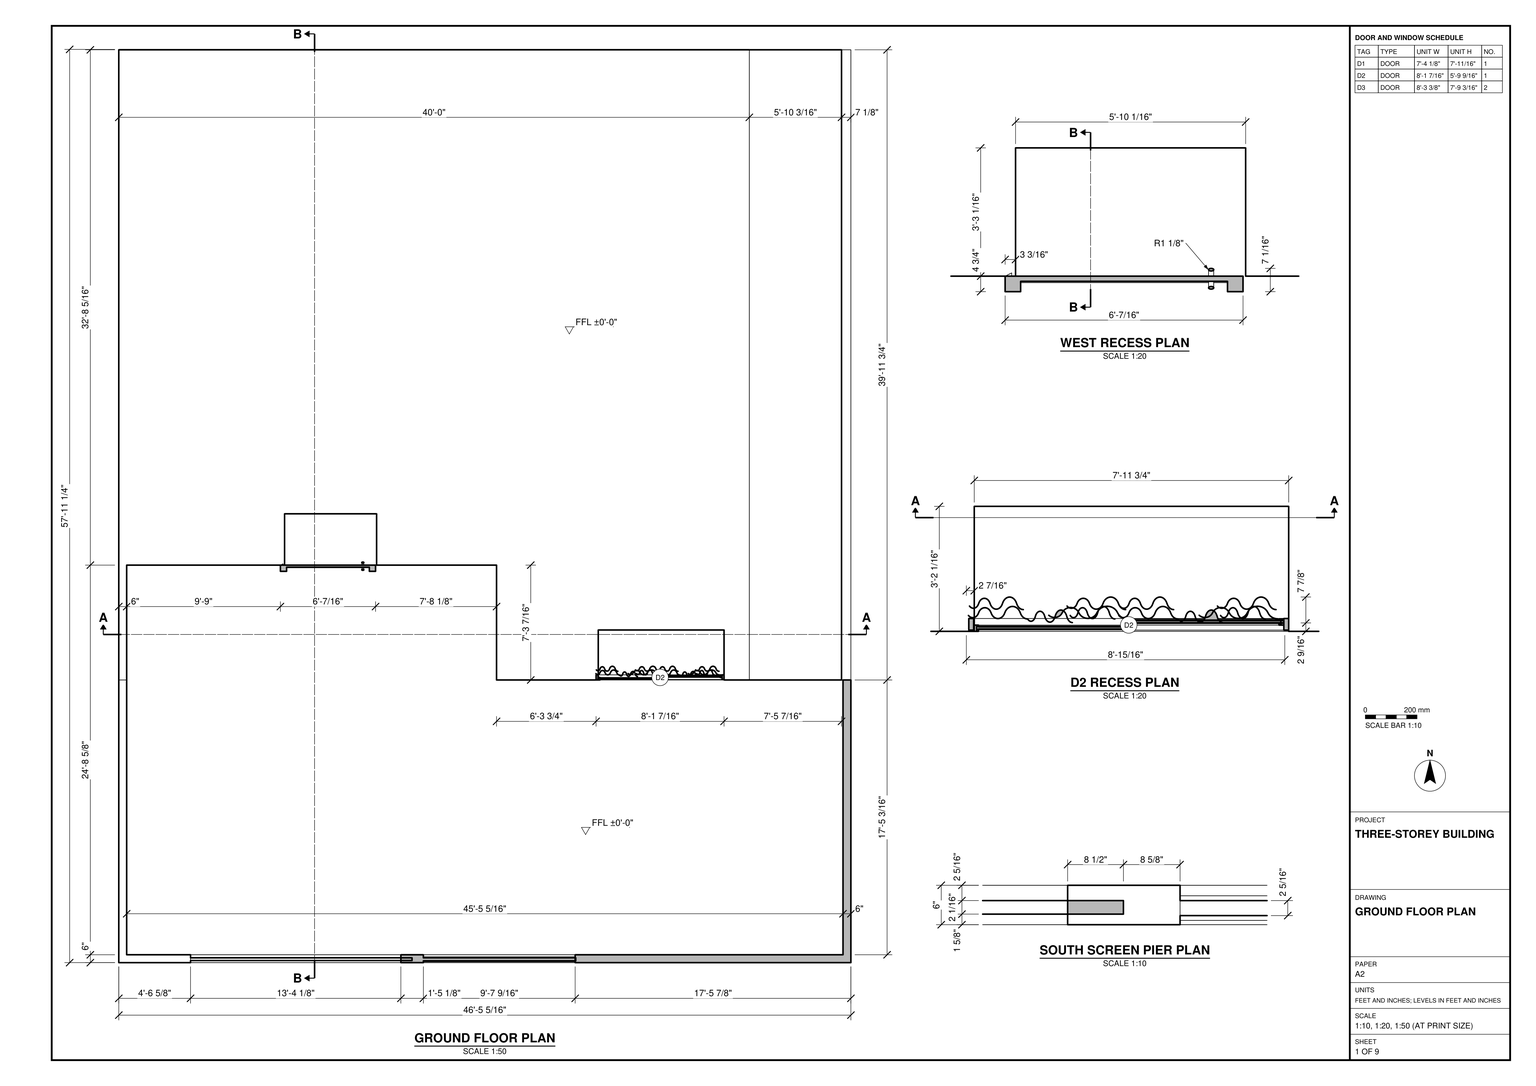
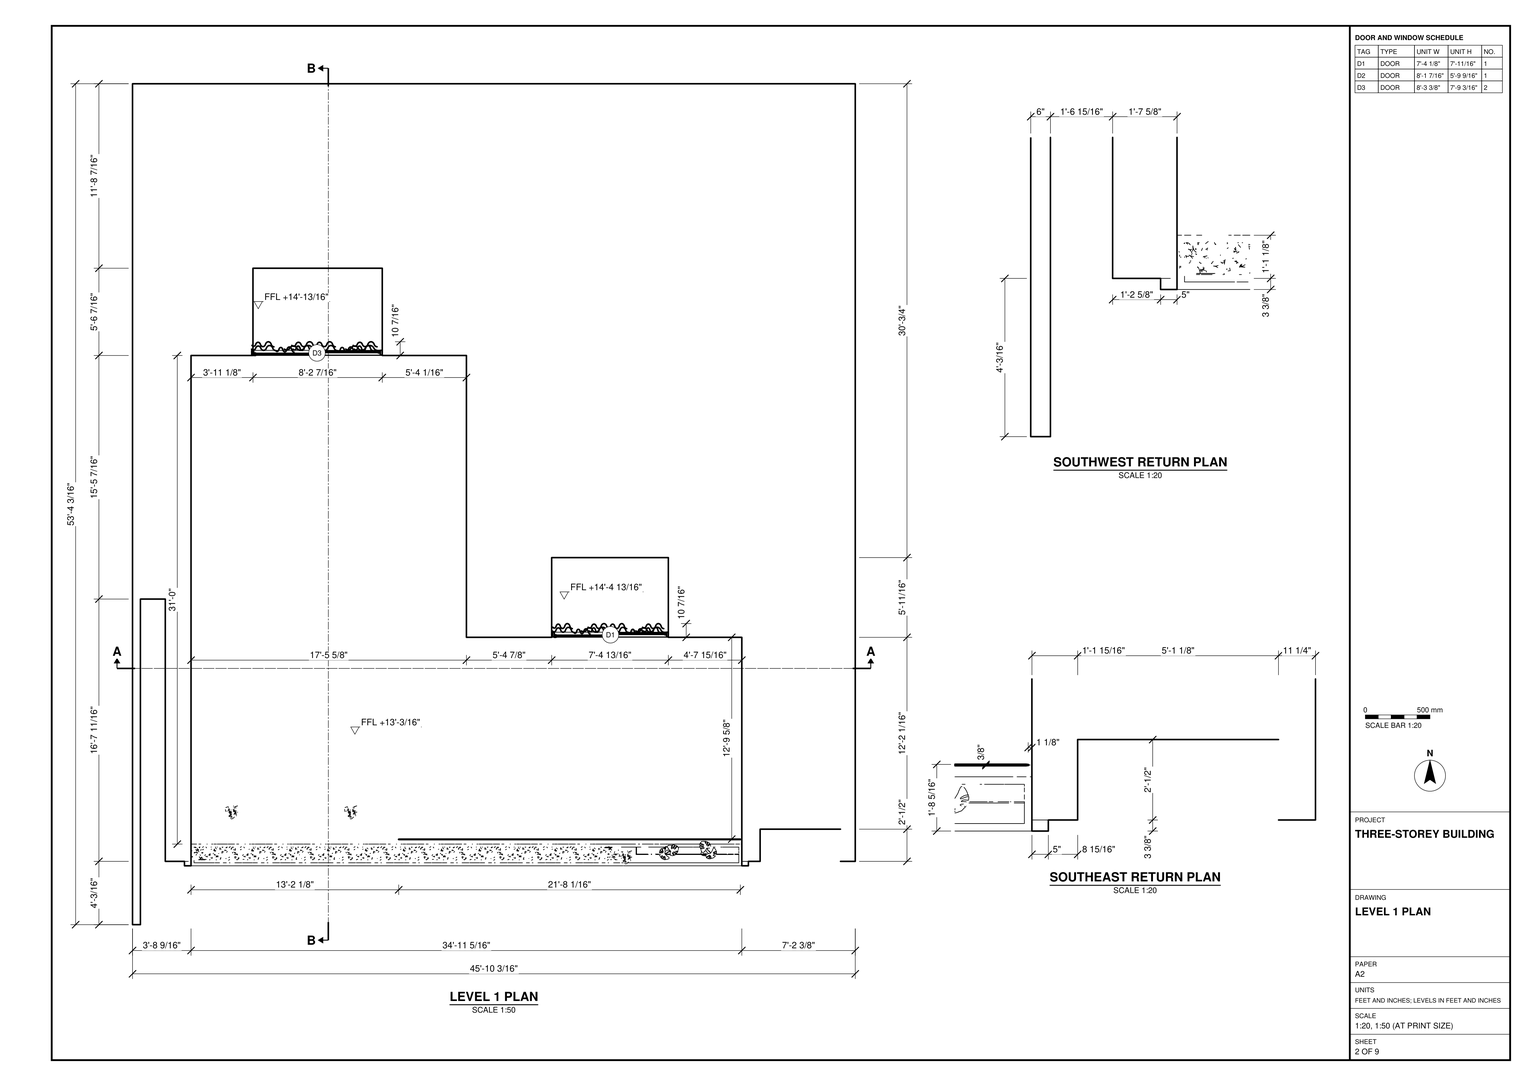
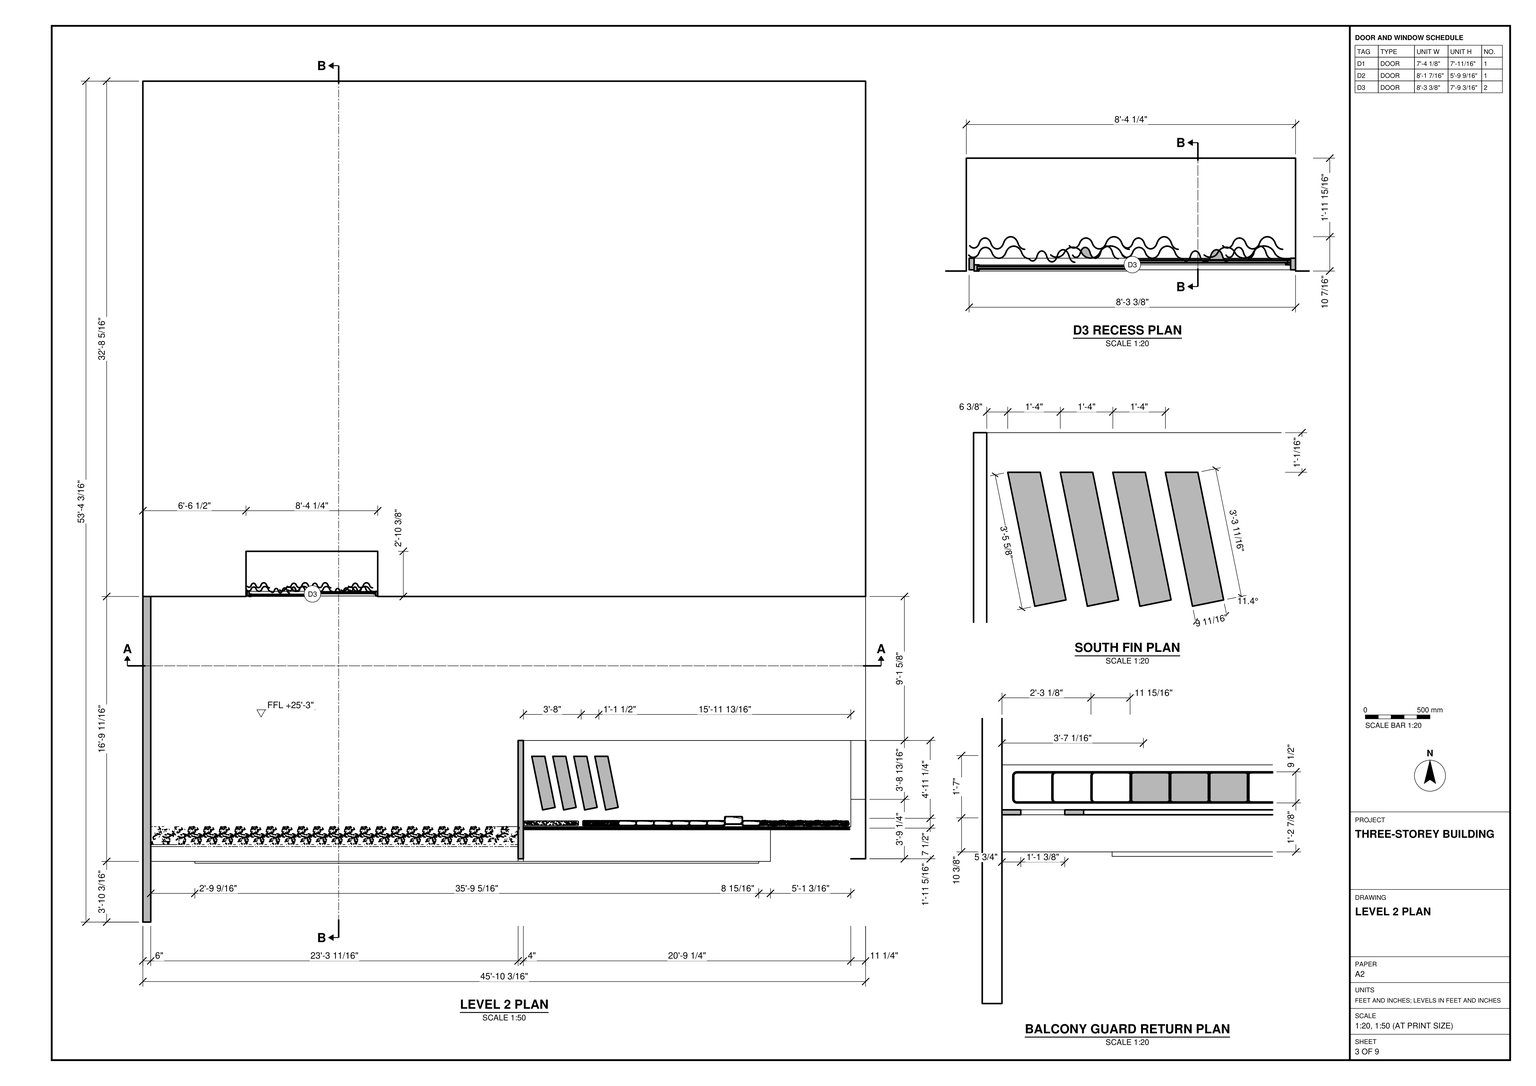
Build the three-storey building shown in task_files/diagram_01.pdf. Work in feet and inches in SketchUp. Orient the model so that the south frontage runs along the X axis. The overall dimensions are 46'-5 5/16" east to west, 57'-11 1/4" north to south and 35'-10 3/8" high. Set the ground floor at ±0'-0", level 1 at +13'-3/16" and level 2 at +25'-3".

Use each floor plan to set out its own walls and slab edges. Follow the wall thicknesses, changes in depth and projecting returns shown on that plan. Complete the roof to the profile shown on the sheets. On the ground floor, distinguish the west recess from the recessed glazed door farther east, and include the pier between the south screen spans. On level 1, place the recessed doors on their respective faces of the stepped wall. Use the enlarged details for the door frames, balcony guards and wall returns. On level 2, include the planting along the south balcony and the angled fins beside the dividing wall.

Keep shell elements such as walls, slabs and roof, and each furniture or joinery piece shown, in separate groups or components. Use components for repeated parts. Decor and loose items, including plants, may be any suitable library components. Save one SketchUp model as output_files/three_storey_building_with_south_balconies.skp.

# SketchUp Ruby script. Lengths in inches.
U = 1.inch
M = Sketchup.active_model
def pt(a) = Geom::Point3d.new(a.map { |v| v * U })
def face(e, loops, mat)
  f = e.add_face(loops[0].map { |a| pt(a) })
  loops[1..].each { |l| e.add_face(l.map { |a| pt(a) }).erase! }
  f.material = f.back_material = mat if mat
  f
end
# faces: each face lists its corners as indices into pts; further lists are holes
def faces(e, pts, list, mat = nil) = list.each { |f| face(e, (f[0].is_a?(Array) ? f : [f]).map { |l| l.map { |i| pts[i] } }, mat) }
# xy, xz, yz: faces in a plane at the given z, y or x. An outline is a flat list of corners, or four numbers for a rectangle; further outlines are holes
def ring(l) = l.size == 4 ? [[l[0], l[1]], [l[2], l[1]], [l[2], l[3]], [l[0], l[3]]] : l.each_slice(2).to_a
def flat(e, list, mat, &to3) = list.each { |f| face(e, (f[0].is_a?(Array) ? f : [f]).map { |l| ring(l).map { |u, v| to3.(u, v) } }, mat) }
def xy(e, z, list, mat = nil) = flat(e, list, mat) { |x, y| [x, y, z] }
def xz(e, y, list, mat = nil) = flat(e, list, mat) { |x, z| [x, y, z] }
def yz(e, x, list, mat = nil) = flat(e, list, mat) { |y, z| [x, y, z] }
def lines(e, pts, list) = list.each { |a, b| e.add_line(pt(pts[a]), pt(pts[b])) }
# prism: a flat outline (further loops are holes) pulled along v
def prism(e, loops, v, mat = nil)
  f = face(e, loops, mat); d = Geom::Vector3d.new(v.map { |x| x * U })
  f.pushpull(f.normal.samedirection?(d) ? d.length : -d.length)
end
def box(e, o, s, mat = nil) = prism(e, [[o, [o[0] + s[0], o[1], o[2]], [o[0] + s[0], o[1] + s[1], o[2]], [o[0], o[1] + s[1], o[2]]]], [0, 0, s[2]], mat)
def at(x, y, z, deg = 0) = Geom::Transformation.translation(pt([x, y, z])) * Geom::Transformation.rotation(ORIGIN, Z_AXIS, deg.degrees)
def axes(o, x, y, z) = Geom::Transformation.new([*x, 0, *y, 0, *z, 0, *pt(o).to_a, 1])
def part(name) = M.definitions.add(name)
# library, detail: a bought-in or finely detailed component or shape, given as its bounding box
def library(name, o, s) = part(name).tap { |d| box(d.entities, o, s) }
def detail(e, o, s) = box(e.add_group.entities, o, s)
def put(e, d, t, mat = nil) = e.add_instance(d, t).tap { |i| i.material = mat if mat }
def group(e, t, mat = nil) = e.add_group.tap { |g| g.transformation = t; g.material = mat if mat }.entities
root = M.entities
M.materials.add("Color_004").color = [142, 142, 142]
M.materials.add("Material__1").color = [51, 42, 44]
M.materials.add("Material__2").color = [97, 132, 37]
M.materials.add("Painted Metal Railing").color = [35, 35, 35]
M.materials.add("Teddy_Paper").color = [237, 237, 189]
M.materials.add("[0135_DarkGray]").color = [81, 81, 81]
M.materials.add("[Color_007]").color = [58, 58, 58]
M.materials.add("[Translucent_Glass_Gray] copy").color = [139, 139, 139]
M.materials["[Translucent_Glass_Gray] copy"].alpha = 0.15
M.materials.add("[Wood Lumber ButtJoined]").color = [164, 152, 112]
M.materials.add("[Wood Veneer 01]1").color = [120, 70, 37]
c1 = part("Post")
box(c1.entities,[-0.75,-0.75,0],[1.5,1.5,34.5],"Painted Metal Railing")
c2 = part("Group43\#1")
box(c2.entities,[-0.75,0,0],[1.5,73.5,1.5],"Painted Metal Railing")
c3 = part("Group46\#2")
box(c3.entities,[-0.75,0.75,0],[1.5,34.5,1.5],"Painted Metal Railing")
c4 = part("Group49\#1")
box(c4.entities,[-0.75,0.75,0],[1.5,34.5,1.5],"Painted Metal Railing")
c5 = part("Group52\#1")
box(c5.entities,[-0.75,0.75,0],[1.5,34.5,1.5],"Painted Metal Railing")
c6 = part("Group55\#1")
box(c6.entities,[-0.75,0.75,0],[1.5,34.5,1.5],"Painted Metal Railing")
c7 = part("Inner Post")
box(c7.entities,[-0.75,-0.75,0],[1.5,1.5,23.5],"Painted Metal Railing")
c8 = part("Group59\#1")
box(c8.entities,[-0.75,0.75,0],[1.5,24.5,1.5],"Painted Metal Railing")
c9 = part("Group62\#1")
box(c9.entities,[-0.75,0.75,0],[1.5,24.5,1.5],"Painted Metal Railing")
c10 = part("Group65\#1")
box(c10.entities,[-0.75,0.75,0],[1.5,24.5,1.5],"Painted Metal Railing")
c11 = part("Inner Posts and Rails\#2")
put(c11.entities,c7,at(0,0,0,90))
put(c11.entities,c7,at(0,26,0,90))
put(c11.entities,c8,at(0,0,4.75))
put(c11.entities,c9,at(0,0,11))
put(c11.entities,c10,at(0,0,17.25))
c12 = part("Group69\#1")
box(c12.entities,[-0.75,0.75,0],[1.5,24.5,1.5],"Painted Metal Railing")
c13 = part("Group72\#1")
box(c13.entities,[-0.75,0.75,0],[1.5,24.5,1.5],"Painted Metal Railing")
c14 = part("Group75\#1")
box(c14.entities,[-0.75,0.75,0],[1.5,24.5,1.5],"Painted Metal Railing")
c15 = part("Inner Posts and Rails\#3")
put(c15.entities,c7,at(0,0,0,90))
put(c15.entities,c7,at(0,26,0,90))
put(c15.entities,c12,at(0,0,4.75))
put(c15.entities,c13,at(0,0,11))
put(c15.entities,c14,at(0,0,17.25))
c16 = part("Railing Assembly 14\#1")
put(c16.entities,c1,at(0,0,0))
put(c16.entities,c1,at(36,0,0))
put(c16.entities,c1,at(72,0,0))
put(c16.entities,c2,at(-0.75,0,34.5,-90))
put(c16.entities,c3,at(0,0,4,-90))
put(c16.entities,c4,at(36,0,4,-90))
put(c16.entities,c5,at(0,0,29,-90))
put(c16.entities,c6,at(36,0,29,-90))
put(c16.entities,c11,at(5,0,5.5,-90))
put(c16.entities,c15,at(41,0,5.5,-90))
c17 = library("Glass Rail",[0,0,0],[2.52,48.73,42.05])
c18 = part("L6T panel")
xy(c18.entities,0,[[0.125,-0.375,27.875,-0.375,28,0,27.875,0.375,0.125,0.375,0,0]],"[Color_007]")
xy(c18.entities,84,[[0.125,-0.375,0,0,0.125,0.375,27.875,0.375,28,0,27.875,-0.375]],"[Color_007]")
xz(c18.entities,-0.375,[[0.125,0,27.875,3.375],[0.125,82.125,27.875,84]],"[Color_007]")
xz(c18.entities,-0.1875,[[0.0625,3.4375,27.9375,82.0625]],"[Translucent_Glass_Gray] copy")
xz(c18.entities,0.1875,[[0.0625,3.4375,27.9375,82.0625]],"[Translucent_Glass_Gray] copy")
xz(c18.entities,0.375,[[0.125,0,27.875,3.375],[0.125,82.125,27.875,84]],"[Color_007]")
yz(c18.entities,0.0625,[[-0.1875,3.4375,0,3.5,0.1875,3.4375,0.1875,82.0625,0,82,-0.1875,82.0625]],"[Translucent_Glass_Gray] copy")
yz(c18.entities,27.9375,[[-0.1875,3.4375,-0.1875,82.0625,0,82,0.1875,82.0625,0.1875,3.4375,0,3.5]],"[Translucent_Glass_Gray] copy")
p = [[0.125,-0.375,0],[0,0,0],[0,0,3.5],[0.0625,-0.1875,3.4375],[0.125,-0.375,3.375],[27.9375,-0.1875,3.4375],
  [28,0,3.5],[28,0,0],[27.875,-0.375,0],[27.875,-0.375,3.375],[0.0625,0.1875,3.4375],[0.125,0.375,0],
  [0.125,0.375,3.375],[27.875,0.375,0],[27.9375,0.1875,3.4375],[27.875,0.375,3.375],[0.0625,0,3.5],[27.9375,0,3.5],
  [0.0625,-0.1875,82.0625],[0,0,82],[0,0,84],[0.125,-0.375,84],[0.125,-0.375,82.125],[27.875,-0.375,84],
  [28,0,84],[28,0,82],[27.9375,-0.1875,82.0625],[27.875,-0.375,82.125],[0.0625,0,82],[27.9375,0,82],
  [0.125,0.375,84],[0.0625,0.1875,82.0625],[0.125,0.375,82.125],[27.9375,0.1875,82.0625],[27.875,0.375,84],[27.875,0.375,82.125]]
faces(c18.entities,p,[[0,1,2,3,4],[5,6,7,8,9],[10,2,1,11,12],[13,7,6,14,15],[4,3,5,9],[2,16,3],[5,3,16,17],[6,5,17],
  [2,16,10],[14,10,16,17],[6,14,17],[12,10,14,15],[18,19,20,21,22],[23,24,25,26,27],[19,18,28],[29,28,18,26],
  [25,29,26],[30,20,19,31,32],[19,31,28],[29,28,31,33],[33,25,24,34,35],[25,29,33],[27,26,18,22],[35,33,31,32]],"[Color_007]")
c19 = part("Group77\#1")
p = [[0,0,0],[0,0,-15.9],[-5.2,0,-15.9],[33.89,-17.6,0],[-33.89,-17.6,0],[33.89,17.6,0],
  [33.89,0,0],[-33.89,17.6,0],[5.2,0,-15.9],[-33.89,0,0],[0,0,-25.75]]
lines(c19.entities,p,[[0,1],[1,2],[3,4],[5,6],[7,5],[1,8],[9,0],[0,6],[8,10],[4,9],[6,3],[2,10],
  [9,7]])
c20 = part("Rectangle Light")
put(c20.entities,c19,at(0,0,0))
c21 = library("Linear planting bed",[-3.03,-4.3,0.15],[92.55,22.69,23.62])
c22 = library("\#1",[-138.85,-135.75,0],[277.7,270.97,9.64])
c23 = library("\#2",[-34.84,-73.35,-33.91],[69.68,146.26,68.31])
c24 = library("\#5",[-4127.85,-1300.75,-2324.72],[5349.84,4521.24,5423.31])
c25 = part("\#3")
put(c25.entities,c24,at(450.18,-1111.4375,0),"Material__2")
c26 = part("12")
put(c26.entities,c22,axes([-49.79,-36.9375,349.64],[0.59279,0,0],[0,0.59279,0],[0,0,0.59279]),"Material__1")
put(c26.entities,c23,axes([-39.24,-18.18,177.19],[1.20819,-2.09264,0],[0,0,2.41638],[2.09264,1.20819,0]))
put(c26.entities,c25,axes([-83.44,-46.04,442.44],[-0.03636,-0.03293,-0.01473],[-0.00083,-0.02391,0.05549],[0.02997,-0.02791,-0.01158]))
c27 = library("3+80",[0,-4.72,-0.01],[36.22,7.09,85.04])
c28 = library("Group\#1",[0,0,0],[100.04,10.85,100.18])
c29 = library("Group8\#1",[-183.25,9.15,0],[25.91,56.79,43.93])
c30 = library("Group13",[-203.48,36.63,0],[29.68,67.31,50.64])
c31 = library("Group8",[-183.25,9.15,0],[25.91,56.79,43.93])
xy(root,-6,[[0,0,557.3125,694.9375],[0,694.9375,480,695.25]])
xy(root,0,[[54.61,0,214.74,6],[231.86,0,347.42,6],[6,6,551.3125,6,551.3125,215.1875,287.5625,215.1875,287.5625,302.625,196.26,302.625,196.26,341.6875,126.2,341.6875,126.2,302.625,6,302.625],[0,215.1875,6,215.1875,6,302.625,126.2,302.625,126.2,341.6875,196.26,341.6875,196.26,302.625,287.5625,302.625,287.5625,215.1875,480,215.1875,480,694.9375,0,694.9375],[480,215.1875,550.1875,694.9375],
  [550.1875,215.1875,557.3125,694.9375],[0,694.9375,480,695.25]])
xy(root,3.51,[[54.61,1.61,218.86,3.67]])
xy(root,7.82,[[54.61,1.61,218.86,3.67]])
xy(root,8.52,[[54.61,1.61,218.55,3.67]])
xy(root,12.83,[[54.61,1.61,218.55,3.67]])
xy(root,13.52,[[54.61,1.61,219.3,3.67]])
xy(root,17.84,[[54.61,1.61,219.3,3.67]])
xy(root,18.53,[[54.61,1.61,216.24,3.67]])
xy(root,22.84,[[54.61,1.61,216.24,3.67]])
xy(root,23.54,[[54.61,1.61,214.74,3.67]])
xy(root,27.85,[[54.61,1.61,214.74,3.67]])
xy(root,28.54,[[54.61,0,214.74,3.67]])
xy(root,28.94,[[365,215.1875,460.75,253.25]])
xy(root,32.86,[[54.61,0,214.74,3.67]])
xy(root,33.55,[[54.61,1.61,216.05,3.67]])
xy(root,37.86,[[54.61,1.61,216.05,3.67]])
xy(root,38.56,[[54.61,1.61,218.55,3.67]])
xy(root,42.87,[[54.61,1.61,218.55,3.67]])
xy(root,43.5625,[[54.61,1.61,223.24,3.67]])
xy(root,47.875,[[54.61,1.61,223.24,3.67]])
xy(root,48.57,[[54.61,1.61,230.3,3.67]])
xy(root,52.88,[[54.61,1.61,230.3,3.67]])
xy(root,53.57,[[54.61,1.61,219.49,3.67]])
xy(root,57.89,[[54.61,1.61,219.49,3.67]])
xy(root,60,[[0,0,54.61,0,54.61,6,6,6,6,94.9375,0,94.9375],[214.74,0,231.86,6],[347.42,0,557.3125,0,557.3125,215.1875,551.3125,215.1875,551.3125,6,347.42,6]])
xy(root,95.5,[[126.2,302.625,196.26,341.6875]])
xy(root,99.13,[[365,215.1875,460.75,253.25]])
xy(root,120,[[0,54.75,6,94.9375]])
xy(root,120,[[24.9375,102.9375,24.9375,302.625,287.5625,302.625,287.5625,215.1875,550.1875,215.1875,550.1875,102.9375,538.9375,102.9375,538.9375,127.4375,477.76,127.4375,477.76,102.9375]],"[Wood Veneer 01]1")
xy(root,151.17,[[463.83,99.5625,468.83,102.9375]])
xy(root,151.17,[[39.54,99.5625,44.54,102.9375],[44.54,99.5625,463.83,102.9375]],"[Wood Veneer 01]1")
xy(root,156.17,[[46.83,101.85,461.54,113.8],[44.54,116.09,463.83,116.09,463.83,273.5,254.1875,273.5,254.1875,488.0625,44.54,488.0625]])
xy(root,163.6,[[[44.54,99.5625,463.83,116.09],[46.83,101.85,461.54,113.8]]],"[Wood Veneer 01]1")
xy(root,168.79,[[91.6875,488.0625,190.125,554.5]])
xy(root,172.8,[[319.08,273.5,407.9,334.1875]])
xy(root,255.86,[[319.08,273.5,407.9,334.1875]])
xy(root,262.29,[[91.6875,488.0625,190.125,554.5]])
xy(root,287.08,[[44.54,99.5625,44.54,488.0625,254.1875,488.0625,254.1875,273.5,463.83,273.5,463.83,99.5625]],"[Wood Veneer 01]1")
xy(root,292.08,[[39.54,99.5625,468.83,102.9375]],"[Wood Veneer 01]1")
xy(root,297,[[6,102.9375,24.9375,127.4375],[6,127.4375,24.9375,302.625]])
xy(root,300.74,[[6,100.9375,289.66,102.9375],[289.66,100.9375,477.76,102.9375]])
xy(root,303,[[6,100.9375,285.66,127.4375],[285.66,100.9375,289.66,102.9375],[289.66,100.9375,477.76,127.4375],[6,127.4375,285.66,127.4375,285.66,193,550.1875,193,550.1875,302.625,178.78,302.625,178.78,337,78.53,337,78.53,302.625,6,302.625]])
xy(root,343.0625,[[[289.66,127.4375,538.9375,193],[352.31,140.14,361.8,142.0625,353.94,180.9375,344.07,180.9375],[336.31,140.14,345.8,142.0625,337.94,180.9375,328.07,180.9375],[320.31,140.14,329.8,142.0625,321.94,180.9375,312.07,180.9375],[304.31,140.14,313.8,142.0625,305.94,180.9375,296.07,180.9375]]])
xy(root,396.45,[[78.53,302.625,178.78,337]])
xy(root,404.75,[[336.31,140.14,328.07,180.9375,337.94,180.9375,345.8,142.0625]])
xy(root,405.3125,[[320.31,140.14,312.07,180.9375,321.94,180.9375,329.8,142.0625]])
xy(root,420,[[0,54.75,6,301.25],[0,301.25,6,302.625],[6,301.25,480,302.625],[0,302.625,480,308.625],[480,302.625,550.1875,308.625],
  [0,308.625,480,694.9375],[480,308.625,550.1875,694.9375]])
xy(root,420,[[285.66,102.9375,550.1875,108.9375],[[285.66,108.9375,550.1875,193],[466.77,113.29,534.09,183.6]]],"Color_004")
xy(root,424.375,[[0,301.25,480,308.625]],"Color_004")
xz(root,0,[[0,-6,557.3125,-6,557.3125,60,347.42,60,347.42,0,231.86,0,231.86,60,214.74,60,214.74,0,54.61,0,54.61,60,0,60],[54.61,28.54,214.74,32.86]])
xz(root,1.61,[[54.61,3.51,218.86,7.82],[54.61,8.52,218.55,12.83],[54.61,13.52,219.3,17.84],[54.61,18.53,216.24,22.84],[54.61,23.54,214.74,27.85],
  [54.61,33.55,216.05,37.86],[54.61,38.56,218.55,42.87],[54.61,43.5625,223.24,47.875],[54.61,48.57,230.3,52.88],[54.61,53.57,219.49,57.89]])
xz(root,3.67,[[54.61,3.51,218.86,7.82],[54.61,8.52,218.55,12.83],[54.61,13.52,219.3,17.84],[54.61,18.53,216.24,22.84],[54.61,23.54,214.74,27.85],
  [54.61,28.54,214.74,32.86],[54.61,33.55,216.05,37.86],[54.61,38.56,218.55,42.87],[54.61,43.5625,223.24,47.875],[54.61,48.57,230.3,52.88],
  [54.61,53.57,219.49,57.89]])
xz(root,6,[[6,0,54.61,60],[214.74,0,231.86,60],[347.42,0,551.3125,60]])
xz(root,54.75,[[0,120,6,420]])
xz(root,94.9375,[[0,60,6,120]])
xz(root,99.5625,[[[39.54,151.17,468.83,292.08],[44.54,163.6,463.83,287.08]]],"[Wood Veneer 01]1")
xz(root,100.9375,[[6,300.74,477.76,303]],"Color_004")
xz(root,101.85,[[46.83,156.17,461.54,163.6]])
xz(root,102.9375,[[538.9375,120,550.1875,120,550.1875,420,285.66,420,285.66,303,289.66,303,289.66,404.7,538.9375,404.7]])
xz(root,102.9375,[[[24.9375,120,477.76,120,477.76,300.74,6,300.74,6,297,24.9375,297],[39.54,151.17,468.83,292.08]]],"[Wood Veneer 01]1")
xz(root,113.29,[[466.77,404.7,534.09,420]])
xz(root,113.8,[[46.83,156.17,461.54,163.6]])
xz(root,116.09,[[44.54,156.17,463.83,163.6]])
xz(root,127.4375,[[477.76,120,538.9375,120,538.9375,343.0625,289.66,343.0625,289.66,303,477.76,303]])
xz(root,180.9375,[[296.07,343.0625,305.94,404.7],[312.07,343.0625,321.94,405.3125],[328.07,343.0625,337.94,404.75],[344.07,343.0625,353.94,404.7]],"[Wood Veneer 01]1")
xz(root,183.6,[[466.77,404.7,534.09,420]])
xz(root,193,[[285.66,303,477.76,303,477.76,343.0625,289.66,343.0625,289.66,354.4375,285.66,354.4375],[477.76,303,538.9375,343.0625],[285.66,354.4375,289.66,354.4375,289.66,404.7,550.1875,404.7,550.1875,420,285.66,420]])
xz(root,215.1875,[[[287.5625,0,550.1875,120],[365,28.94,460.75,99.13]],[551.3125,0,557.3125,60]])
xz(root,253.25,[[365,28.94,460.75,99.13]])
xz(root,273.5,[[[254.1875,156.17,463.83,287.08],[319.08,172.8,407.9,255.86]]])
xz(root,301.25,[[0,420,480,424.375]],"Color_004")
xz(root,302.625,[[0,295.4375,6,420],[6,295.4375,24.9375,297],[6,303,78.53,303,78.53,396.45,178.78,396.45,178.78,303,480,303,480,420,6,420],[480,303,550.1875,420]])
xz(root,302.625,[[6,0,126.2,0,126.2,95.5,196.26,95.5,196.26,0,287.5625,0,287.5625,120,24.9375,120,24.9375,295.4375,6,295.4375]],"[Wood Veneer 01]1")
xz(root,308.625,[[0,420,6,424.375],[6,420,480,424.375]])
xz(root,334.1875,[[319.08,172.8,407.9,255.86]])
xz(root,337,[[78.53,303,178.78,396.45]])
xz(root,341.6875,[[126.2,0,196.26,95.5]])
xz(root,488.0625,[[[44.54,156.17,254.1875,287.08],[91.6875,168.79,190.125,262.29]]])
xz(root,554.5,[[91.6875,168.79,190.125,262.29]])
xz(root,694.9375,[[480,-6,557.3125,0],[0,0,480,120],[480,0,550.1875,120],[0,120,480,295.4375],[480,120,550.1875,295.4375],
  [0,295.4375,480,420],[480,295.4375,550.1875,420]])
xz(root,695.25,[[0,-6,480,0]])
yz(root,0,[[0,-6,0,60,94.9375,60,94.9375,0,694.9375,0,694.9375,-6],[694.9375,-6,695.25,0],[94.9375,0,94.9375,120,54.75,120,54.75,420,302.625,420,302.625,295.4375,694.9375,295.4375,694.9375,120,215.1875,120,215.1875,0],[215.1875,0,694.9375,120],[302.625,295.4375,694.9375,420]])
yz(root,0,[[301.25,420,308.625,424.375]],"Color_004")
yz(root,6,[[6,0,94.9375,60]])
yz(root,6,[[54.75,240,54.75,420,302.625,420,302.625,303,100.9375,303,100.9375,300.74,102.9375,300.74,102.9375,297,302.625,297,302.625,240]],"Teddy_Paper")
yz(root,6,[[94.9375,0,302.625,0,302.625,240,54.75,240,54.75,120,94.9375,120]],"[Wood Lumber ButtJoined]")
yz(root,24.9375,[[102.9375,120,302.625,297]],"[Wood Lumber ButtJoined]")
yz(root,39.54,[[99.5625,287.08,102.9375,292.08]])
yz(root,39.54,[[99.5625,151.17,102.9375,156.17],[99.5625,156.17,102.9375,287.08]],"[Wood Lumber ButtJoined]")
yz(root,44.54,[[116.09,156.17,488.0625,156.17,488.0625,287.08,99.5625,287.08,99.5625,163.6,116.09,163.6]])
yz(root,46.83,[[101.85,156.17,113.8,163.6]])
yz(root,54.61,[[[0,0,6,0,6,60,0,60,0,32.86,3.67,32.86,3.67,28.54,0,28.54],[1.61,53.57,3.67,57.89],[1.61,48.57,3.67,52.88],[1.61,43.5625,3.67,47.875],[1.61,38.56,3.67,42.87],[1.61,33.55,3.67,37.86],[1.61,23.54,3.67,27.85],[1.61,18.53,3.67,22.84],[1.61,13.52,3.67,17.84],[1.61,8.52,3.67,12.83],[1.61,3.51,3.67,7.82]]])
yz(root,78.53,[[302.625,303,337,396.45]])
yz(root,91.6875,[[488.0625,168.79,554.5,262.29]])
yz(root,126.2,[[302.625,0,341.6875,95.5]])
yz(root,178.78,[[302.625,303,337,396.45]])
yz(root,190.125,[[488.0625,168.79,554.5,262.29]])
yz(root,196.26,[[302.625,0,341.6875,95.5]])
yz(root,214.74,[[[0,0,0,28.54,3.67,28.54,3.67,32.86,0,32.86,0,60,6,60,6,0],[1.61,23.54,3.67,27.85]]])
yz(root,216.05,[[1.61,33.55,3.67,37.86]])
yz(root,216.24,[[1.61,18.53,3.67,22.84]])
yz(root,218.55,[[1.61,8.52,3.67,12.83],[1.61,38.56,3.67,42.87]])
yz(root,218.86,[[1.61,3.51,3.67,7.82]])
yz(root,219.3,[[1.61,13.52,3.67,17.84]])
yz(root,219.49,[[1.61,53.57,3.67,57.89]])
yz(root,223.24,[[1.61,43.5625,3.67,47.875]])
yz(root,230.3,[[1.61,48.57,3.67,52.88]])
yz(root,231.86,[[[0,0,6,60],[2.53,51.41,2.04,51.48,1.59,51.66,1.2,51.96,0.9,52.35,0.72,52.8,0.65,53.29,0.72,53.77,0.9,54.22,1.2,54.61,1.59,54.91,2.04,55.1,2.53,55.16,3.01,55.1,3.46,54.91,3.85,54.61,4.15,54.22,4.34,53.77,4.4,53.29,4.34,52.8,4.15,52.35,3.85,51.96,3.46,51.66,3.01,51.48],[2.53,43.9,2.04,43.97,1.59,44.15,1.2,44.45,0.9,44.84,0.72,45.29,0.65,45.78,0.72,46.26,0.9,46.71,1.2,47.1,1.59,47.4,2.04,47.59,2.53,47.65,3.01,47.59,3.46,47.4,3.85,47.1,4.15,46.71,4.34,46.26,4.4,45.78,4.34,45.29,4.15,44.84,3.85,44.45,3.46,44.15,3.01,43.97],[2.53,36.39,2.04,36.46,1.59,36.64,1.2,36.94,0.9,37.33,0.72,37.78,0.65,38.27,0.72,38.75,0.9,39.2,1.2,39.59,1.59,39.89,2.04,40.08,2.53,40.14,3.01,40.08,3.46,39.89,3.85,39.59,4.15,39.2,4.34,38.75,4.4,38.27,4.34,37.78,4.15,37.33,3.85,36.94,3.46,36.64,3.01,36.46],[2.53,28.88,2.04,28.94,1.59,29.13,1.2,29.43,0.9,29.82,0.72,30.27,0.65,30.76,0.72,31.24,0.9,31.69,1.2,32.08,1.59,32.38,2.04,32.57,2.53,32.63,3.01,32.57,3.46,32.38,3.85,32.08,4.15,31.69,4.34,31.24,4.4,30.76,4.34,30.27,4.15,29.82,3.85,29.43,3.46,29.13,3.01,28.94],[2.53,21.37,2.04,21.43,1.59,21.62,1.2,21.92,0.9,22.31,0.72,22.76,0.65,23.25,0.72,23.73,0.9,24.18,1.2,24.57,1.59,24.87,2.04,25.06,2.53,25.12,3.01,25.06,3.46,24.87,3.85,24.57,4.15,24.18,4.34,23.73,4.4,23.25,4.34,22.76,4.15,22.31,3.85,21.92,3.46,21.62,3.01,21.43],[2.53,13.86,2.04,13.92,1.59,14.11,1.2,14.41,0.9,14.8,0.72,15.25,0.65,15.74,0.72,16.22,0.9,16.67,1.2,17.0625,1.59,17.36,2.04,17.55,2.53,17.61,3.01,17.55,3.46,17.36,3.85,17.0625,4.15,16.67,4.34,16.22,4.4,15.74,4.34,15.25,4.15,14.8,3.85,14.41,3.46,14.11,3.01,13.92],[2.53,6.35,2.04,6.41,1.59,6.6,1.2,6.9,0.9,7.29,0.72,7.74,0.65,8.22,0.72,8.71,0.9,9.16,1.2,9.55,1.59,9.85,2.04,10.04,2.53,10.1,3.01,10.04,3.46,9.85,3.85,9.55,4.15,9.16,4.34,8.71,4.4,8.22,4.34,7.74,4.15,7.29,3.85,6.9,3.46,6.6,3.01,6.41]]])
yz(root,254.1875,[[273.5,156.17,488.0625,287.08]])
yz(root,285.66,[[102.9375,303,193,420]])
yz(root,287.5625,[[215.1875,0,302.625,120]])
yz(root,289.66,[[102.9375,303,127.4375,303,127.4375,343.0625,193,343.0625,193,404.7,102.9375,404.7]])
yz(root,319.08,[[273.5,172.8,334.1875,255.86]])
yz(root,347.42,[[[0,0,6,60],[2.53,6.35,3.01,6.41,3.46,6.6,3.85,6.9,4.15,7.29,4.34,7.74,4.4,8.22,4.34,8.71,4.15,9.16,3.85,9.55,3.46,9.85,3.01,10.04,2.53,10.1,2.04,10.04,1.59,9.85,1.2,9.55,0.9,9.16,0.72,8.71,0.65,8.22,0.72,7.74,0.9,7.29,1.2,6.9,1.59,6.6,2.04,6.41]]])
yz(root,347.86,[[2.53,43.9,3.01,43.97,3.46,44.15,3.85,44.45,4.15,44.84,4.34,45.29,4.4,45.78,4.34,46.26,4.15,46.71,3.85,47.1,3.46,47.4,3.01,47.59,2.53,47.65,2.04,47.59,1.59,47.4,1.2,47.1,0.9,46.71,0.72,46.26,0.65,45.78,0.72,45.29,0.9,44.84,1.2,44.45,1.59,44.15,2.04,43.97]])
yz(root,348.48,[[2.53,13.86,3.01,13.92,3.46,14.11,3.85,14.41,4.15,14.8,4.34,15.25,4.4,15.74,4.34,16.22,4.15,16.67,3.85,17.0625,3.46,17.36,3.01,17.55,2.53,17.61,2.04,17.55,1.59,17.36,1.2,17.0625,0.9,16.67,0.72,16.22,0.65,15.74,0.72,15.25,0.9,14.8,1.2,14.41,1.59,14.11,2.04,13.92]])
yz(root,351.73,[[2.53,51.41,3.01,51.48,3.46,51.66,3.85,51.96,4.15,52.35,4.34,52.8,4.4,53.29,4.34,53.77,4.15,54.22,3.85,54.61,3.46,54.91,3.01,55.1,2.53,55.16,2.04,55.1,1.59,54.91,1.2,54.61,0.9,54.22,0.72,53.77,0.65,53.29,0.72,52.8,0.9,52.35,1.2,51.96,1.59,51.66,2.04,51.48]])
yz(root,354.17,[[2.53,36.39,3.01,36.46,3.46,36.64,3.85,36.94,4.15,37.33,4.34,37.78,4.4,38.27,4.34,38.75,4.15,39.2,3.85,39.59,3.46,39.89,3.01,40.08,2.53,40.14,2.04,40.08,1.59,39.89,1.2,39.59,0.9,39.2,0.72,38.75,0.65,38.27,0.72,37.78,0.9,37.33,1.2,36.94,1.59,36.64,2.04,36.46]])
yz(root,355.92,[[2.53,21.37,3.01,21.43,3.46,21.62,3.85,21.92,4.15,22.31,4.34,22.76,4.4,23.25,4.34,23.73,4.15,24.18,3.85,24.57,3.46,24.87,3.01,25.06,2.53,25.12,2.04,25.06,1.59,24.87,1.2,24.57,0.9,24.18,0.72,23.73,0.65,23.25,0.72,22.76,0.9,22.31,1.2,21.92,1.59,21.62,2.04,21.43]])
yz(root,365,[[215.1875,28.94,253.25,99.13]])
yz(root,403.98,[[2.53,28.88,3.01,28.94,3.46,29.13,3.85,29.43,4.15,29.82,4.34,30.27,4.4,30.76,4.34,31.24,4.15,31.69,3.85,32.08,3.46,32.38,3.01,32.57,2.53,32.63,2.04,32.57,1.59,32.38,1.2,32.08,0.9,31.69,0.72,31.24,0.65,30.76,0.72,30.27,0.9,29.82,1.2,29.43,1.59,29.13,2.04,28.94]])
yz(root,407.9,[[273.5,172.8,334.1875,255.86]])
yz(root,460.75,[[215.1875,28.94,253.25,99.13]])
yz(root,461.54,[[101.85,156.17,113.8,163.6]])
yz(root,463.83,[[116.09,156.17,116.09,163.6,99.5625,163.6,99.5625,287.08,273.5,287.08,273.5,156.17]])
yz(root,466.77,[[113.29,404.7,183.6,420]])
yz(root,468.83,[[99.5625,151.17,102.9375,156.17],[99.5625,156.17,102.9375,292.08]])
yz(root,477.76,[[102.9375,120,127.4375,120,127.4375,303,100.9375,303,100.9375,300.74,102.9375,300.74]])
yz(root,480,[[694.9375,-6,695.25,0],[301.25,420,308.625,424.375]])
yz(root,534.09,[[113.29,404.7,183.6,420]])
yz(root,550.1875,[[215.1875,0,215.1875,120,102.9375,120,102.9375,404.7,193,404.7,193,303,302.625,303,302.625,420,694.9375,420,694.9375,0],[102.9375,404.7,193,420]])
yz(root,551.3125,[[6,0,215.1875,60]])
yz(root,557.3125,[[0,-6,694.9375,-6,694.9375,0,215.1875,0,215.1875,60,0,60]])
p = [[231.86,2.04,6.41],[231.86,2.53,6.35],[347.42,2.53,6.35],[347.42,2.04,6.41],[231.86,3.01,6.41],[347.42,3.01,6.41],
  [231.86,1.59,6.6],[347.42,1.59,6.6],[231.86,3.46,6.6],[347.42,3.46,6.6],[231.86,1.2,6.9],[347.42,1.2,6.9],
  [231.86,3.85,6.9],[347.42,3.85,6.9],[231.86,0.9,7.29],[347.42,0.9,7.29],[231.86,4.15,7.29],[347.42,4.15,7.29],
  [231.86,0.72,7.74],[347.42,0.72,7.74],[231.86,4.34,7.74],[347.42,4.34,7.74],[231.86,0.65,8.22],[347.42,0.65,8.22],
  [231.86,4.4,8.22],[347.42,4.4,8.22],[231.86,0.72,8.71],[347.42,0.72,8.71],[231.86,4.34,8.71],[347.42,4.34,8.71],
  [231.86,0.9,9.16],[347.42,0.9,9.16],[231.86,4.15,9.16],[347.42,4.15,9.16],[231.86,1.2,9.55],[347.42,1.2,9.55],
  [231.86,3.85,9.55],[347.42,3.85,9.55],[231.86,1.59,9.85],[347.42,1.59,9.85],[231.86,3.46,9.85],[347.42,3.46,9.85],
  [231.86,2.04,10.04],[347.42,2.04,10.04],[231.86,3.01,10.04],[347.42,3.01,10.04],[231.86,2.53,10.1],[347.42,2.53,10.1],
  [231.86,1.59,14.11],[231.86,2.04,13.92],[348.48,2.04,13.92],[348.48,1.59,14.11],[231.86,2.53,13.86],[348.48,2.53,13.86],
  [231.86,3.01,13.92],[348.48,3.01,13.92],[231.86,3.46,14.11],[348.48,3.46,14.11],[231.86,1.2,14.41],[348.48,1.2,14.41],
  [231.86,3.85,14.41],[348.48,3.85,14.41],[231.86,0.9,14.8],[348.48,0.9,14.8],[231.86,4.15,14.8],[348.48,4.15,14.8],
  [231.86,0.72,15.25],[348.48,0.72,15.25],[231.86,4.34,15.25],[348.48,4.34,15.25],[231.86,0.65,15.74],[348.48,0.65,15.74],
  [231.86,4.4,15.74],[348.48,4.4,15.74],[231.86,0.72,16.22],[348.48,0.72,16.22],[231.86,4.34,16.22],[348.48,4.34,16.22],
  [231.86,0.9,16.67],[348.48,0.9,16.67],[231.86,4.15,16.67],[348.48,4.15,16.67],[231.86,1.2,17.0625],[348.48,1.2,17.0625],
  [231.86,3.85,17.0625],[348.48,3.85,17.0625],[231.86,1.59,17.36],[348.48,1.59,17.36],[231.86,3.46,17.36],[348.48,3.46,17.36],
  [231.86,2.04,17.55],[348.48,2.04,17.55],[231.86,3.01,17.55],[348.48,3.01,17.55],[231.86,2.53,17.61],[348.48,2.53,17.61],
  [231.86,1.59,21.62],[231.86,2.04,21.43],[355.92,2.04,21.43],[355.92,1.59,21.62],[231.86,2.53,21.37],[355.92,2.53,21.37],
  [231.86,3.01,21.43],[355.92,3.01,21.43],[231.86,3.46,21.62],[355.92,3.46,21.62],[231.86,1.2,21.92],[355.92,1.2,21.92],
  [231.86,3.85,21.92],[355.92,3.85,21.92],[231.86,0.9,22.31],[355.92,0.9,22.31],[231.86,4.15,22.31],[355.92,4.15,22.31],
  [231.86,0.72,22.76],[355.92,0.72,22.76],[231.86,4.34,22.76],[355.92,4.34,22.76],[231.86,0.65,23.25],[355.92,0.65,23.25],
  [231.86,4.4,23.25],[355.92,4.4,23.25],[231.86,0.72,23.73],[355.92,0.72,23.73],[231.86,4.34,23.73],[355.92,4.34,23.73],
  [231.86,0.9,24.18],[355.92,0.9,24.18],[231.86,4.15,24.18],[355.92,4.15,24.18],[231.86,1.2,24.57],[355.92,1.2,24.57],
  [231.86,3.85,24.57],[355.92,3.85,24.57],[231.86,1.59,24.87],[355.92,1.59,24.87],[231.86,3.46,24.87],[355.92,3.46,24.87],
  [231.86,2.04,25.06],[355.92,2.04,25.06],[231.86,3.01,25.06],[355.92,3.01,25.06],[231.86,2.53,25.12],[355.92,2.53,25.12],
  [231.86,1.59,29.13],[231.86,2.04,28.94],[403.98,2.04,28.94],[403.98,1.59,29.13],[231.86,2.53,28.88],[403.98,2.53,28.88],
  [231.86,3.01,28.94],[403.98,3.01,28.94],[231.86,3.46,29.13],[403.98,3.46,29.13],[231.86,1.2,29.43],[403.98,1.2,29.43],
  [231.86,3.85,29.43],[403.98,3.85,29.43],[231.86,0.9,29.82],[403.98,0.9,29.82],[231.86,4.15,29.82],[403.98,4.15,29.82],
  [231.86,0.72,30.27],[403.98,0.72,30.27],[231.86,4.34,30.27],[403.98,4.34,30.27],[231.86,0.65,30.76],[403.98,0.65,30.76],
  [231.86,4.4,30.76],[403.98,4.4,30.76],[231.86,0.72,31.24],[403.98,0.72,31.24],[231.86,4.34,31.24],[403.98,4.34,31.24],
  [231.86,0.9,31.69],[403.98,0.9,31.69],[231.86,4.15,31.69],[403.98,4.15,31.69],[231.86,1.2,32.08],[403.98,1.2,32.08],
  [231.86,3.85,32.08],[403.98,3.85,32.08],[231.86,1.59,32.38],[403.98,1.59,32.38],[231.86,3.46,32.38],[403.98,3.46,32.38],
  [231.86,2.04,32.57],[403.98,2.04,32.57],[231.86,3.01,32.57],[403.98,3.01,32.57],[231.86,2.53,32.63],[403.98,2.53,32.63],
  [231.86,2.04,36.46],[231.86,2.53,36.39],[354.17,2.53,36.39],[354.17,2.04,36.46],[231.86,3.01,36.46],[354.17,3.01,36.46],
  [231.86,1.59,36.64],[354.17,1.59,36.64],[231.86,3.46,36.64],[354.17,3.46,36.64],[231.86,1.2,36.94],[354.17,1.2,36.94],
  [231.86,3.85,36.94],[354.17,3.85,36.94],[231.86,0.9,37.33],[354.17,0.9,37.33],[231.86,4.15,37.33],[354.17,4.15,37.33],
  [231.86,0.72,37.78],[354.17,0.72,37.78],[231.86,4.34,37.78],[354.17,4.34,37.78],[231.86,0.65,38.27],[354.17,0.65,38.27],
  [231.86,4.4,38.27],[354.17,4.4,38.27],[231.86,0.72,38.75],[354.17,0.72,38.75],[231.86,4.34,38.75],[354.17,4.34,38.75],
  [231.86,0.9,39.2],[354.17,0.9,39.2],[231.86,4.15,39.2],[354.17,4.15,39.2],[231.86,1.2,39.59],[354.17,1.2,39.59],
  [231.86,3.85,39.59],[354.17,3.85,39.59],[231.86,1.59,39.89],[354.17,1.59,39.89],[231.86,3.46,39.89],[354.17,3.46,39.89],
  [231.86,2.04,40.08],[354.17,2.04,40.08],[231.86,3.01,40.08],[354.17,3.01,40.08],[231.86,2.53,40.14],[354.17,2.53,40.14],
  [231.86,2.04,43.97],[231.86,2.53,43.9],[347.86,2.53,43.9],[347.86,2.04,43.97],[231.86,3.01,43.97],[347.86,3.01,43.97],
  [231.86,1.59,44.15],[347.86,1.59,44.15],[231.86,3.46,44.15],[347.86,3.46,44.15],[231.86,1.2,44.45],[347.86,1.2,44.45],
  [231.86,3.85,44.45],[347.86,3.85,44.45],[231.86,0.9,44.84],[347.86,0.9,44.84],[231.86,4.15,44.84],[347.86,4.15,44.84],
  [231.86,0.72,45.29],[347.86,0.72,45.29],[231.86,4.34,45.29],[347.86,4.34,45.29],[231.86,0.65,45.78],[347.86,0.65,45.78],
  [231.86,4.4,45.78],[347.86,4.4,45.78],[231.86,0.72,46.26],[347.86,0.72,46.26],[231.86,4.34,46.26],[347.86,4.34,46.26],
  [231.86,0.9,46.71],[347.86,0.9,46.71],[231.86,4.15,46.71],[347.86,4.15,46.71],[231.86,1.2,47.1],[347.86,1.2,47.1],
  [231.86,3.85,47.1],[347.86,3.85,47.1],[231.86,1.59,47.4],[347.86,1.59,47.4],[231.86,3.46,47.4],[347.86,3.46,47.4],
  [231.86,2.04,47.59],[347.86,2.04,47.59],[231.86,3.01,47.59],[347.86,3.01,47.59],[231.86,2.53,47.65],[347.86,2.53,47.65],
  [231.86,2.04,51.48],[231.86,2.53,51.41],[351.73,2.53,51.41],[351.73,2.04,51.48],[231.86,3.01,51.48],[351.73,3.01,51.48],
  [231.86,1.59,51.66],[351.73,1.59,51.66],[231.86,3.46,51.66],[351.73,3.46,51.66],[231.86,1.2,51.96],[351.73,1.2,51.96],
  [231.86,3.85,51.96],[351.73,3.85,51.96],[231.86,0.9,52.35],[351.73,0.9,52.35],[231.86,4.15,52.35],[351.73,4.15,52.35],
  [231.86,0.72,52.8],[351.73,0.72,52.8],[231.86,4.34,52.8],[351.73,4.34,52.8],[231.86,0.65,53.29],[351.73,0.65,53.29],
  [231.86,4.4,53.29],[351.73,4.4,53.29],[231.86,0.72,53.77],[351.73,0.72,53.77],[231.86,4.34,53.77],[351.73,4.34,53.77],
  [231.86,0.9,54.22],[351.73,0.9,54.22],[231.86,4.15,54.22],[351.73,4.15,54.22],[231.86,1.2,54.61],[351.73,1.2,54.61],
  [231.86,3.85,54.61],[351.73,3.85,54.61],[231.86,1.59,54.91],[351.73,1.59,54.91],[231.86,3.46,54.91],[351.73,3.46,54.91],
  [231.86,2.04,55.1],[351.73,2.04,55.1],[231.86,3.01,55.1],[351.73,3.01,55.1],[231.86,2.53,55.16],[351.73,2.53,55.16],
  [304.31,140.14,343.0625],[296.07,180.9375,343.0625],[296.07,180.9375,404.7],[304.31,140.14,404.7],[313.8,142.0625,343.0625],[313.8,142.0625,404.7],
  [320.31,140.14,343.0625],[312.07,180.9375,343.0625],[312.07,180.9375,405.3125],[320.31,140.14,405.3125],[329.8,142.0625,343.0625],[329.8,142.0625,405.3125],
  [336.31,140.14,343.0625],[328.07,180.9375,343.0625],[328.07,180.9375,404.75],[336.31,140.14,404.75],[345.8,142.0625,343.0625],[345.8,142.0625,404.75],
  [352.31,140.14,343.0625],[344.07,180.9375,343.0625],[344.07,180.9375,404.7],[352.31,140.14,404.7],[361.8,142.0625,343.0625],[361.8,142.0625,404.7],
  [305.94,180.9375,343.0625],[305.94,180.9375,404.7],[321.94,180.9375,343.0625],[321.94,180.9375,405.3125],[337.94,180.9375,343.0625],[337.94,180.9375,404.75],
  [353.94,180.9375,343.0625],[353.94,180.9375,404.7],[0,215.1875,120],[6,215.1875,120],[24.9375,302.625,295.4375],[480,302.625,295.4375],
  [538.9375,148.1875,303],[550.1875,148.1875,303],[538.9375,148.1875,343.0625],[538.9375,193,303]]
faces(root,p,[[0,1,2,3],[1,4,5,2],[6,0,3,7],[4,8,9,5],[10,6,7,11],[8,12,13,9],[14,10,11,15],[12,16,17,13],
  [18,14,15,19],[16,20,21,17],[22,18,19,23],[20,24,25,21],[26,22,23,27],[24,28,29,25],[30,26,27,31],[28,32,33,29],
  [34,30,31,35],[32,36,37,33],[38,34,35,39],[36,40,41,37],[42,38,39,43],[40,44,45,41],[46,42,43,47],[44,46,47,45],
  [48,49,50,51],[49,52,53,50],[52,54,55,53],[54,56,57,55],[58,48,51,59],[56,60,61,57],[62,58,59,63],[60,64,65,61],
  [66,62,63,67],[64,68,69,65],[70,66,67,71],[68,72,73,69],[74,70,71,75],[72,76,77,73],[78,74,75,79],[76,80,81,77],
  [82,78,79,83],[80,84,85,81],[86,82,83,87],[84,88,89,85],[90,86,87,91],[88,92,93,89],[94,90,91,95],[92,94,95,93],
  [96,97,98,99],[97,100,101,98],[100,102,103,101],[102,104,105,103],[106,96,99,107],[104,108,109,105],[110,106,107,111],[108,112,113,109],
  [114,110,111,115],[112,116,117,113],[118,114,115,119],[116,120,121,117],[122,118,119,123],[120,124,125,121],[126,122,123,127],[124,128,129,125],
  [130,126,127,131],[128,132,133,129],[134,130,131,135],[132,136,137,133],[138,134,135,139],[136,140,141,137],[142,138,139,143],[140,142,143,141],
  [144,145,146,147],[145,148,149,146],[148,150,151,149],[150,152,153,151],[154,144,147,155],[152,156,157,153],[158,154,155,159],[156,160,161,157],
  [162,158,159,163],[160,164,165,161],[166,162,163,167],[164,168,169,165],[170,166,167,171],[168,172,173,169],[174,170,171,175],[172,176,177,173],
  [178,174,175,179],[176,180,181,177],[182,178,179,183],[180,184,185,181],[186,182,183,187],[184,188,189,185],[190,186,187,191],[188,190,191,189],
  [192,193,194,195],[193,196,197,194],[198,192,195,199],[196,200,201,197],[202,198,199,203],[200,204,205,201],[206,202,203,207],[204,208,209,205],
  [210,206,207,211],[208,212,213,209],[214,210,211,215],[212,216,217,213],[218,214,215,219],[216,220,221,217],[222,218,219,223],[220,224,225,221],
  [226,222,223,227],[224,228,229,225],[230,226,227,231],[228,232,233,229],[234,230,231,235],[232,236,237,233],[238,234,235,239],[236,238,239,237],
  [240,241,242,243],[241,244,245,242],[246,240,243,247],[244,248,249,245],[250,246,247,251],[248,252,253,249],[254,250,251,255],[252,256,257,253],
  [258,254,255,259],[256,260,261,257],[262,258,259,263],[260,264,265,261],[266,262,263,267],[264,268,269,265],[270,266,267,271],[268,272,273,269],
  [274,270,271,275],[272,276,277,273],[278,274,275,279],[276,280,281,277],[282,278,279,283],[280,284,285,281],[286,282,283,287],[284,286,287,285],
  [288,289,290,291],[289,292,293,290],[294,288,291,295],[292,296,297,293],[298,294,295,299],[296,300,301,297],[302,298,299,303],[300,304,305,301],
  [306,302,303,307],[304,308,309,305],[310,306,307,311],[308,312,313,309],[314,310,311,315],[312,316,317,313],[318,314,315,319],[316,320,321,317],
  [322,318,319,323],[320,324,325,321],[326,322,323,327],[324,328,329,325],[330,326,327,331],[328,332,333,329],[334,330,331,335],[332,334,335,333]],"[0135_DarkGray]")
faces(root,p,[[336,337,338,339],[340,336,339,341],[342,343,344,345],[346,342,345,347],[348,349,350,351],[352,348,351,353],[354,355,356,357],[358,354,357,359],
  [360,340,341,361],[362,346,347,363],[364,352,353,365],[366,358,359,367]],"[Wood Veneer 01]1")
lines(root,p,[[368,369],[370,371],[372,373],[372,374],[372,375]])
put(root,c16,axes([8.87,112.99,303],[3.8253,0,0],[0,1,0],[0,0,1]))
put(root,c17,axes([289.66,127.4375,343.0625],[0,-1,0],[5.12535,0,0],[0,0,0.52]))
put(root,c18,axes([202.05,119.6875,156.17],[9.33,0,0],[0,1,0],[0,0,1.61807]))
put(root,c20,axes([144.16,554.49,225.92],[0.8272,0,0],[0,0,-0.7832],[0,0.88,0]))
put(root,c20,axes([372.68,334.1875,215.11],[0.8272,0,0],[0,0,-0.7832],[0,0.88,0]))
put(root,c21,at(379.3125,103.86,156.17))
put(root,c26,axes([169.18,142.21,156.17],[0.0583,0,0],[0,0.0583,0],[0,0,0.0583]))
put(root,c26,axes([378.47,107.98,156.23],[0.0583,0,0],[0,0.0583,0],[0,0,0.0583]))
put(root,c26,axes([78.44,142.21,156.17],[0.0583,0,0],[0,0.0583,0],[0,0,0.0583]))
put(root,c27,axes([123.02,302.62,0],[2,0,0],[0,1,0],[0,0,1.13]))
put(root,c28,axes([319.08,273.5,172.8],[0.88781,0,0],[0,0.96371,0],[0,0,0.85326]))
put(root,c28,axes([89.96,488.0625,168.79],[1.0013,0,0],[0,0.96371,0],[0,0,0.93859]))
put(root,c29,axes([519.8125,80.61,343.0625],[0,-0.29,0],[0.29,0,0],[0,0,0.29]))
put(root,c30,axes([306.93,-11.67,154.26],[0,-0.64,0],[0.64,0,0],[0,0,0.64]))
put(root,c30,axes([278.09,-11.67,153.95],[0,-0.64,0],[0.64,0,0],[0,0,0.64]))
put(root,c30,axes([249.26,-11.67,153.64],[0,-0.64,0],[0.64,0,0],[0,0,0.64]))
put(root,c30,axes([220.43,-11.67,153.33],[0,-0.64,0],[0.64,0,0],[0,0,0.64]))
put(root,c30,axes([191.6,-11.67,153.02],[0,-0.64,0],[0.64,0,0],[0,0,0.64]))
put(root,c30,axes([162.76,-11.67,152.71],[0,-0.64,0],[0.64,0,0],[0,0,0.64]))
put(root,c30,axes([133.93,-11.67,152.4],[0,-0.64,0],[0.64,0,0],[0,0,0.64]))
put(root,c30,axes([105.1,-11.67,152.09],[0,-0.64,0],[0.64,0,0],[0,0,0.64]))
put(root,c30,axes([76.26,-11.67,151.79],[0,-0.64,0],[0.64,0,0],[0,0,0.64]))
put(root,c30,axes([47.43,-11.67,151.48],[0,-0.64,0],[0.64,0,0],[0,0,0.64]))
put(root,c30,axes([18.6,-11.67,151.17],[0,-0.64,0],[0.64,0,0],[0,0,0.64]))
put(root,c29,axes([506.33,80.61,343.0625],[0,-0.29,0],[0.29,0,0],[0,0,0.29]))
put(root,c29,axes([492.84,80.61,343.0625],[0,-0.29,0],[0.29,0,0],[0,0,0.29]))
put(root,c29,axes([479.35,80.61,343.0625],[0,-0.29,0],[0.29,0,0],[0,0,0.29]))
put(root,c29,axes([465.86,80.61,343.0625],[0,-0.29,0],[0.29,0,0],[0,0,0.29]))
put(root,c29,axes([452.375,80.61,343.0625],[0,-0.29,0],[0.29,0,0],[0,0,0.4582]))
put(root,c29,axes([438.89,54.61,343.0625],[0,-0.4553,0],[0.29,0,0],[0,0,0.58]))
put(root,c31,axes([425.4,80.61,343.0625],[0,-0.29,0],[0.29,0,0],[0,0,0.4727]))
put(root,c29,axes([411.91,80.61,343.0625],[0,-0.29,0],[0.29,0,0],[0,0,0.4756]))
put(root,c29,axes([398.43,80.61,343.0625],[0,-0.29,0],[0.29,0,0],[0,0,0.4466]))
put(root,c29,axes([384.9375,80.61,343.0625],[0,-0.29,0],[0.29,0,0],[0,0,0.4669]))
put(root,c29,axes([371.45,80.61,343.0625],[0,-0.29,0],[0.29,0,0],[0,0,0.4582]))
put(root,c29,axes([357.96,80.61,343.0625],[0,-0.29,0],[0.29,0,0],[0,0,0.435]))
put(root,c29,axes([344.48,80.61,343.0625],[0,-0.29,0],[0.29,0,0],[0,0,0.4002]))
put(root,c29,axes([330.99,80.61,343.0625],[0,-0.29,0],[0.29,0,0],[0,0,0.4031]))
put(root,c29,axes([277.45,80.61,343.0625],[0,-0.29,0],[0.89728,0,0],[0,0,0.3596]))
put(root,c28,axes([362.59,215.1875,28.94],[0.98127,0,0],[0,0.96371,0],[0,0,0.70059]),"[Wood Veneer 01]1")
put(root,c28,axes([78.62,302.625,303],[1.0013,0,0],[0,0.96371,0],[0,0,0.93859]))
put(root,c30,axes([220.71,0.06,303],[0,-0.64,0],[0.64,0,0],[0,0,1.0432]))
put(root,c30,axes([208.8,0.06,303],[0,-0.64,0],[0.64,0,0],[0,0,1.0432]))
put(root,c30,axes([196.89,0.06,303],[0,-0.64,0],[0.64,0,0],[0,0,1.0432]))
put(root,c30,axes([184.98,0.06,303],[0,-0.64,0],[0.64,0,0],[0,0,1.0432]))
put(root,c30,axes([173.08,0.06,303],[0,-0.64,0],[0.64,0,0],[0,0,1.0432]))
put(root,c30,axes([161.17,0.06,303],[0,-0.64,0],[0.64,0,0],[0,0,1.0432]))
put(root,c30,axes([149.26,0.06,303],[0,-0.64,0],[0.64,0,0],[0,0,1.0432]))
put(root,c30,axes([137.35,0.06,303],[0,-0.64,0],[0.64,0,0],[0,0,1.0432]))
put(root,c30,axes([125.45,0.06,303],[0,-0.64,0],[0.64,0,0],[0,0,1.0432]))
put(root,c30,axes([113.54,0.06,303],[0,-0.64,0],[0.64,0,0],[0,0,1.0432]))
put(root,c30,axes([101.63,0.06,303],[0,-0.64,0],[0.64,0,0],[0,0,1.0432]))
put(root,c30,axes([89.72,0.06,303],[0,-0.64,0],[0.64,0,0],[0,0,1.0432]))
put(root,c30,axes([77.82,0.06,303],[0,-0.64,0],[0.64,0,0],[0,0,1.0432]))
put(root,c30,axes([65.91,0.06,303],[0,-0.64,0],[0.64,0,0],[0,0,1.0432]))
put(root,c30,axes([54,0.06,303],[0,-0.64,0],[0.64,0,0],[0,0,1.0432]))
put(root,c30,axes([42.09,0.06,303],[0,-0.64,0],[0.64,0,0],[0,0,1.0432]))
put(root,c30,axes([30.19,0.06,303],[0,-0.64,0],[0.64,0,0],[0,0,1.0432]))
put(root,c30,axes([18.28,0.06,303],[0,-0.64,0],[0.64,0,0],[0,0,1.0432]))
put(root,c30,axes([6.37,0.06,303],[0,-0.64,0],[0.64,0,0],[0,0,1.0432]))
put(root,c30,axes([-5.54,0.06,303],[0,-0.64,0],[0.64,0,0],[0,0,1.0432]))
put(root,c30,axes([-17.44,0.06,303],[0,-0.64,0],[0.64,0,0],[0,0,1.0432]))
